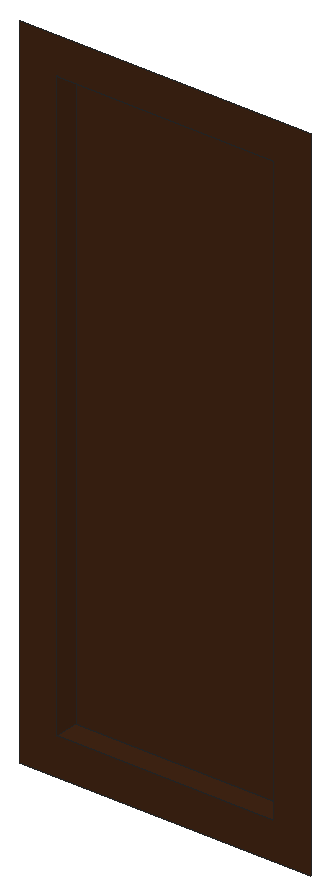
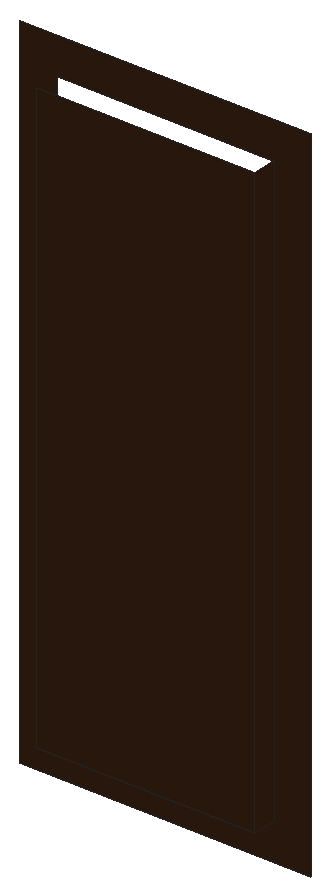
# SketchUp Ruby script. Lengths in inches.
U = 1.inch
M = Sketchup.active_model
def pt(a) = Geom::Point3d.new(a.map { |v| v * U })
def face(e, loops, mat)
  f = e.add_face(loops[0].map { |a| pt(a) })
  loops[1..].each { |l| e.add_face(l.map { |a| pt(a) }).erase! }
  f.material = f.back_material = mat if mat
  f
end
# faces: each face lists its corners as indices into pts; further lists are holes
def faces(e, pts, list, mat = nil) = list.each { |f| face(e, (f[0].is_a?(Array) ? f : [f]).map { |l| l.map { |i| pts[i] } }, mat) }
# xy, xz, yz: faces in a plane at the given z, y or x. An outline is a flat list of corners, or four numbers for a rectangle; further outlines are holes
def ring(l) = l.size == 4 ? [[l[0], l[1]], [l[2], l[1]], [l[2], l[3]], [l[0], l[3]]] : l.each_slice(2).to_a
def flat(e, list, mat, &to3) = list.each { |f| face(e, (f[0].is_a?(Array) ? f : [f]).map { |l| ring(l).map { |u, v| to3.(u, v) } }, mat) }
def xy(e, z, list, mat = nil) = flat(e, list, mat) { |x, y| [x, y, z] }
def xz(e, y, list, mat = nil) = flat(e, list, mat) { |x, z| [x, y, z] }
def yz(e, x, list, mat = nil) = flat(e, list, mat) { |y, z| [x, y, z] }
def lines(e, pts, list) = list.each { |a, b| e.add_line(pt(pts[a]), pt(pts[b])) }
# prism: a flat outline (further loops are holes) pulled along v
def prism(e, loops, v, mat = nil)
  f = face(e, loops, mat); d = Geom::Vector3d.new(v.map { |x| x * U })
  f.pushpull(f.normal.samedirection?(d) ? d.length : -d.length)
end
def box(e, o, s, mat = nil) = prism(e, [[o, [o[0] + s[0], o[1], o[2]], [o[0] + s[0], o[1] + s[1], o[2]], [o[0], o[1] + s[1], o[2]]]], [0, 0, s[2]], mat)
def at(x, y, z, deg = 0) = Geom::Transformation.translation(pt([x, y, z])) * Geom::Transformation.rotation(ORIGIN, Z_AXIS, deg.degrees)
def axes(o, x, y, z) = Geom::Transformation.new([*x, 0, *y, 0, *z, 0, *pt(o).to_a, 1])
def part(name) = M.definitions.add(name)
# library, detail: a bought-in or finely detailed component or shape, given as its bounding box
def library(name, o, s) = part(name).tap { |d| box(d.entities, o, s) }
def detail(e, o, s) = box(e.add_group.entities, o, s)
def put(e, d, t, mat = nil) = e.add_instance(d, t).tap { |i| i.material = mat if mat }
def group(e, t, mat = nil) = e.add_group.tap { |g| g.transformation = t; g.material = mat if mat }.entities
root = M.entities
M.materials.add("[Wood Veneer 01]").color = [66, 38, 20]
xy(root,135.37,[[209.83,244.48,239.03,247.79]],"[Wood Veneer 01]")
xz(root,244.48,[[[204.93,130.46,243.93,219.72],[209.83,135.37,239.03,214.82]]],"[Wood Veneer 01]")
xz(root,247.79,[[209.83,135.37,239.03,214.82]],"[Wood Veneer 01]")
yz(root,209.83,[[244.48,135.37,247.79,214.82]],"[Wood Veneer 01]")
